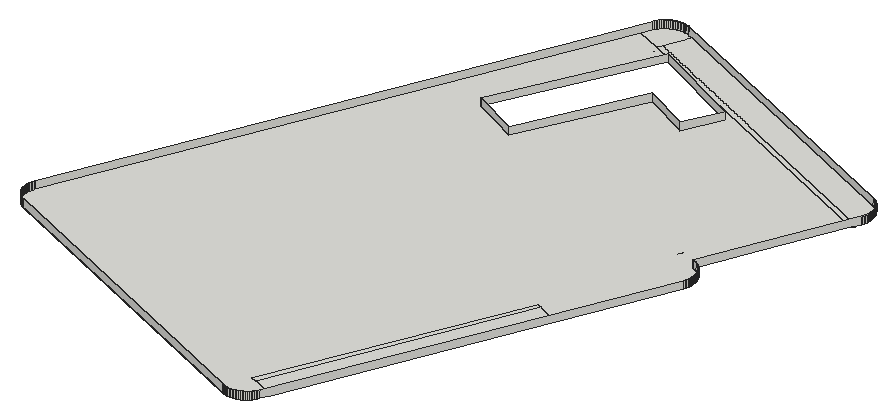
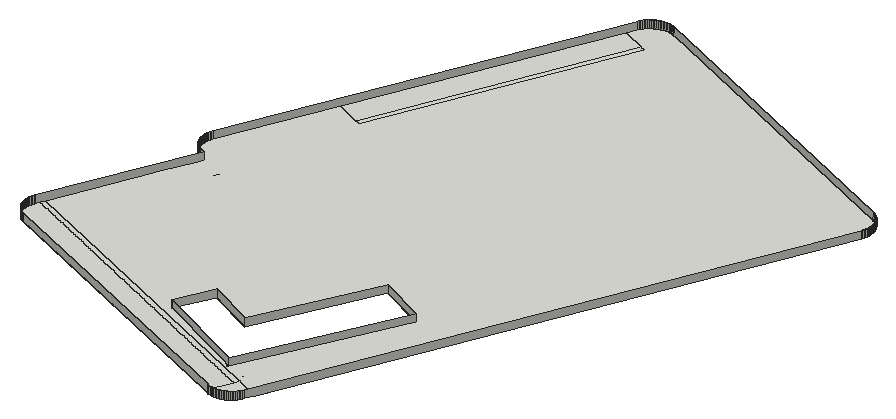
# SketchUp Ruby script. Lengths in inches.
U = 1.inch
M = Sketchup.active_model
def pt(a) = Geom::Point3d.new(a.map { |v| v * U })
def face(e, loops, mat)
  f = e.add_face(loops[0].map { |a| pt(a) })
  loops[1..].each { |l| e.add_face(l.map { |a| pt(a) }).erase! }
  f.material = f.back_material = mat if mat
  f
end
# faces: each face lists its corners as indices into pts; further lists are holes
def faces(e, pts, list, mat = nil) = list.each { |f| face(e, (f[0].is_a?(Array) ? f : [f]).map { |l| l.map { |i| pts[i] } }, mat) }
# xy, xz, yz: faces in a plane at the given z, y or x. An outline is a flat list of corners, or four numbers for a rectangle; further outlines are holes
def ring(l) = l.size == 4 ? [[l[0], l[1]], [l[2], l[1]], [l[2], l[3]], [l[0], l[3]]] : l.each_slice(2).to_a
def flat(e, list, mat, &to3) = list.each { |f| face(e, (f[0].is_a?(Array) ? f : [f]).map { |l| ring(l).map { |u, v| to3.(u, v) } }, mat) }
def xy(e, z, list, mat = nil) = flat(e, list, mat) { |x, y| [x, y, z] }
def xz(e, y, list, mat = nil) = flat(e, list, mat) { |x, z| [x, y, z] }
def yz(e, x, list, mat = nil) = flat(e, list, mat) { |y, z| [x, y, z] }
def lines(e, pts, list) = list.each { |a, b| e.add_line(pt(pts[a]), pt(pts[b])) }
# prism: a flat outline (further loops are holes) pulled along v
def prism(e, loops, v, mat = nil)
  f = face(e, loops, mat); d = Geom::Vector3d.new(v.map { |x| x * U })
  f.pushpull(f.normal.samedirection?(d) ? d.length : -d.length)
end
def box(e, o, s, mat = nil) = prism(e, [[o, [o[0] + s[0], o[1], o[2]], [o[0] + s[0], o[1] + s[1], o[2]], [o[0], o[1] + s[1], o[2]]]], [0, 0, s[2]], mat)
def at(x, y, z, deg = 0) = Geom::Transformation.translation(pt([x, y, z])) * Geom::Transformation.rotation(ORIGIN, Z_AXIS, deg.degrees)
def axes(o, x, y, z) = Geom::Transformation.new([*x, 0, *y, 0, *z, 0, *pt(o).to_a, 1])
def part(name) = M.definitions.add(name)
# library, detail: a bought-in or finely detailed component or shape, given as its bounding box
def library(name, o, s) = part(name).tap { |d| box(d.entities, o, s) }
def detail(e, o, s) = box(e.add_group.entities, o, s)
def put(e, d, t, mat = nil) = e.add_instance(d, t).tap { |i| i.material = mat if mat }
def group(e, t, mat = nil) = e.add_group.tap { |g| g.transformation = t; g.material = mat if mat }.entities
root = M.entities
xy(root,306,[[841.44,516.19,840.14,516.26,838.84,516.41,837.55,516.64,836.28,516.96,835.03,517.37,833.82,517.85,548.6875,642.03,547.51,642.59,546.36,643.23,545.26,643.94,544.21,644.73,543.22,645.57,542.28,646.49,541.4,647.46,540.59,648.48,539.85,649.56,539.18,650.68,538.58,651.85,538.0625,653.05,537.62,654.28,537.26,655.54,536.99,656.82,536.8,658.12,536.7,659.42,536.68,660.73,536.74,662.04,536.9,663.34,537.13,664.625,537.45,665.89,537.85,667.14,538.34,668.36,737.58,1125.82,759.58,1116.24,781.77,1106.57,780.33,1103.61,714.3125,967.65,757.25,946.81,807.7,1050.72,850.64,1029.87,866.2,1061.92,780.33,1103.61,781.77,1106.57,1037.38,995.25,1022.45,960.98,1002.39,914.92,999.84,909.07,987.46,880.65,985.47,876.0625,989.14,874.47,990.32,873.91,991.46,873.27,992.56,872.56,993.61,871.78,994.61,870.93,995.54,870.01,996.42,869.04,997.23,868.02,997.98,866.94,998.65,865.82,999.24,864.65,999.76,863.45,1000.2,862.22,1000.56,860.96,1000.83,859.68,1001.02,858.38,1001.13,857.08,1001.15,855.77,1001.08,854.46,1000.93,853.16,1000.69,851.875,1000.37,850.61,999.97,849.36,999.49,848.14,957.56,751.88,935.56,761.46,930.97,763.46,837.14,548.01,841.72,546.01,863.72,536.43,860.14,528.2,859.58,527.02,858.94,525.875,858.23,524.78,857.45,523.73,856.6,522.73,855.6875,521.79,854.72,520.91,853.69,520.1,852.61,519.36,851.49,518.6875,850.32,518.09,849.125,517.57,847.89,517.14,846.63,516.78,845.35,516.5,844.06,516.3125,842.75,516.21],[863.72,536.43,841.72,546.01,935.56,761.46,957.56,751.88],[841.72,546.01,837.14,548.01,930.97,763.46,935.56,761.46],[1037.38,995.25,781.77,1106.57,759.58,1116.24,761.77,1120.74,1039.375,999.83],[1037.38,995.25,1039.5625,999.75,1039.375,999.83],
  [1039.375,999.83,761.77,1120.74,771.35,1142.74,1030.62,1029.82,1031.8,1029.26,1032.95,1028.625,1034.04,1027.91,1035.09,1027.13,1036.09,1026.28,1037.03,1025.37,1037.91,1024.4,1038.72,1023.375,1039.46,1022.3,1040.13,1021.17,1040.73,1020.01,1041.25,1018.81,1041.6875,1017.57,1042.04,1016.31,1042.32,1015.03,1042.51,1013.74,1042.61,1012.44,1042.63,1011.125,1042.57,1009.82,1042.41,1008.52,1042.18,1007.23,1041.86,1005.96,1041.45,1004.72,1040.97,1003.5],[759.58,1116.24,737.58,1125.82,741.17,1134.07,741.73,1135.26,742.37,1136.4,743.08,1137.5,743.86,1138.55,744.71,1139.54,745.625,1140.48,746.59,1141.36,747.62,1142.17,748.7,1142.92,749.82,1143.59,750.99,1144.18,752.1875,1144.7,753.42,1145.14,754.68,1145.5,755.96,1145.77,757.26,1145.96,758.56,1146.07,759.87,1146.08,761.18,1146.02,762.48,1145.87,763.76,1145.63,765.03,1145.31,766.28,1144.91,767.49,1144.42,771.35,1142.74,761.77,1120.74]])
p = [[841.44,516.19,306],[841.44,516.19,312.91],[840.14,516.26,312.91],[840.14,516.26,306],[842.75,516.21,306],[842.75,516.21,312.91],
  [844.06,516.3125,306],[844.06,516.3125,312.91],[838.84,516.41,312.91],[838.84,516.41,306],[845.35,516.5,306],[845.35,516.5,312.91],
  [837.55,516.64,312.91],[837.55,516.64,306],[846.63,516.78,306],[846.63,516.78,312.91],[836.28,516.96,312.91],[836.28,516.96,306],
  [847.89,517.14,306],[847.89,517.14,312.91],[835.03,517.37,312.91],[835.03,517.37,306],[849.125,517.57,306],[849.125,517.57,312.91],
  [833.82,517.85,312.91],[833.82,517.85,306],[850.32,518.09,306],[850.32,518.09,312.91],[548.6875,642.03,312.91],[548.6875,642.03,306],
  [851.49,518.6875,306],[851.49,518.6875,312.91],[852.61,519.36,306],[852.61,519.36,312.91],[853.69,520.1,306],[853.69,520.1,312.91],
  [854.72,520.91,306],[854.72,520.91,312.91],[855.6875,521.79,306],[855.6875,521.79,312.91],[856.6,522.73,306],[856.6,522.73,312.91],
  [857.45,523.73,306],[857.45,523.73,312.91],[858.23,524.78,306],[858.23,524.78,312.91],[858.94,525.875,306],[858.94,525.875,312.91],
  [859.58,527.02,306],[859.58,527.02,312.91],[860.14,528.2,306],[860.14,528.2,312.91],[957.56,751.88,306],[999.49,848.14,306],
  [999.49,848.14,312.91],[863.72,536.43,306],[547.51,642.59,312.91],[547.51,642.59,306],[546.36,643.23,312.91],[546.36,643.23,306],
  [545.26,643.94,312.91],[545.26,643.94,306],[544.21,644.73,312.91],[544.21,644.73,306],[543.22,645.57,312.91],[543.22,645.57,306],
  [542.28,646.49,312.91],[542.28,646.49,306],[541.4,647.46,312.91],[541.4,647.46,306],[540.59,648.48,312.91],[540.59,648.48,306],
  [539.85,649.56,312.91],[539.85,649.56,306],[539.18,650.68,312.91],[539.18,650.68,306],[538.58,651.85,312.91],[538.58,651.85,306],
  [538.0625,653.05,312.91],[538.0625,653.05,306],[537.62,654.28,312.91],[537.62,654.28,306],[537.26,655.54,312.91],[537.26,655.54,306],
  [536.99,656.82,312.91],[536.99,656.82,306],[536.8,658.12,312.91],[536.8,658.12,306],[536.7,659.42,312.91],[536.7,659.42,306],
  [536.68,660.73,312.91],[536.68,660.73,306],[536.74,662.04,312.91],[536.74,662.04,306],[536.9,663.34,312.91],[536.9,663.34,306],
  [537.13,664.625,312.91],[537.13,664.625,306],[537.45,665.89,312.91],[537.45,665.89,306],[537.85,667.14,312.91],[537.85,667.14,306],
  [538.34,668.36,312.91],[538.34,668.36,306],[741.17,1134.07,312.91],[741.17,1134.07,306],[737.58,1125.82,306],[999.97,849.36,306],
  [999.97,849.36,312.91],[1000.37,850.61,306],[1000.37,850.61,312.91],[1000.69,851.875,306],[1000.69,851.875,312.91],[1000.93,853.16,306],
  [1000.93,853.16,312.91],[1001.08,854.46,306],[1001.08,854.46,312.91],[1001.15,855.77,306],[1001.15,855.77,312.91],[1001.13,857.08,306],
  [1001.13,857.08,312.91],[1001.02,858.38,306],[1001.02,858.38,312.91],[1000.83,859.68,306],[1000.83,859.68,312.91],[1000.56,860.96,306],
  [1000.56,860.96,312.91],[1000.2,862.22,306],[1000.2,862.22,312.91],[999.76,863.45,306],[999.76,863.45,312.91],[999.24,864.65,306],
  [999.24,864.65,312.91],[998.65,865.82,306],[998.65,865.82,312.91],[997.98,866.94,306],[997.98,866.94,312.91],[997.23,868.02,306],
  [997.23,868.02,312.91],[996.42,869.04,306],[996.42,869.04,312.91],[995.54,870.01,306],[995.54,870.01,312.91],[994.61,870.93,306],
  [994.61,870.93,312.91],[993.61,871.78,306],[993.61,871.78,312.91],[992.56,872.56,306],[992.56,872.56,312.91],[991.46,873.27,306],
  [991.46,873.27,312.91],[990.32,873.91,306],[990.32,873.91,312.91],[989.14,874.47,306],[989.14,874.47,312.91],[985.47,876.0625,312.91],
  [985.47,876.0625,306],[1039.375,999.83,306],[1040.97,1003.5,306],[1040.97,1003.5,312.91],[987.46,880.65,306],[999.84,909.07,306],
  [1002.39,914.92,306],[1022.45,960.98,306],[1037.38,995.25,306],[714.3125,967.65,312.91],[757.25,946.81,312.91],[757.25,946.81,306],
  [714.3125,967.65,306],[807.7,1050.72,312.91],[807.7,1050.72,306],[780.33,1103.61,312.91],[780.33,1103.61,306],[1041.45,1004.72,306],
  [1041.45,1004.72,312.91],[1041.86,1005.96,306],[1041.86,1005.96,312.91],[1042.18,1007.23,306],[1042.18,1007.23,312.91],[1042.41,1008.52,306],
  [1042.41,1008.52,312.91],[1042.57,1009.82,306],[1042.57,1009.82,312.91],[1042.63,1011.125,306],[1042.63,1011.125,312.91],[1042.61,1012.44,306],
  [1042.61,1012.44,312.91],[1042.51,1013.74,306],[1042.51,1013.74,312.91],[1042.32,1015.03,306],[1042.32,1015.03,312.91],[1042.04,1016.31,306],
  [1042.04,1016.31,312.91],[1041.6875,1017.57,306],[1041.6875,1017.57,312.91],[1041.25,1018.81,306],[1041.25,1018.81,312.91],[1040.73,1020.01,306],
  [1040.73,1020.01,312.91],[1040.13,1021.17,306],[1040.13,1021.17,312.91],[1039.46,1022.3,306],[1039.46,1022.3,312.91],[1038.72,1023.375,306],
  [1038.72,1023.375,312.91],[1037.91,1024.4,306],[1037.91,1024.4,312.91],[1037.03,1025.37,306],[1037.03,1025.37,312.91],[1036.09,1026.28,306],
  [1036.09,1026.28,312.91],[1035.09,1027.13,306],[1035.09,1027.13,312.91],[1034.04,1027.91,306],[1034.04,1027.91,312.91],[1032.95,1028.625,306],
  [1032.95,1028.625,312.91],[1031.8,1029.26,306],[1031.8,1029.26,312.91],[1030.62,1029.82,306],[1030.62,1029.82,312.91],[767.49,1144.42,312.91],
  [771.35,1142.74,306],[767.49,1144.42,306],[850.64,1029.87,312.91],[850.64,1029.87,306],[866.2,1061.92,306],[866.2,1061.92,312.91],
  [741.73,1135.26,312.91],[741.73,1135.26,306],[742.37,1136.4,312.91],[742.37,1136.4,306],[743.08,1137.5,312.91],[743.08,1137.5,306],
  [743.86,1138.55,312.91],[743.86,1138.55,306],[744.71,1139.54,312.91],[744.71,1139.54,306],[745.625,1140.48,312.91],[745.625,1140.48,306],
  [746.59,1141.36,312.91],[746.59,1141.36,306],[747.62,1142.17,312.91],[747.62,1142.17,306],[748.7,1142.92,312.91],[748.7,1142.92,306],
  [749.82,1143.59,312.91],[749.82,1143.59,306],[750.99,1144.18,312.91],[750.99,1144.18,306],[752.1875,1144.7,312.91],[752.1875,1144.7,306],
  [766.28,1144.91,306],[766.28,1144.91,312.91],[753.42,1145.14,312.91],[753.42,1145.14,306],[765.03,1145.31,306],[765.03,1145.31,312.91],
  [754.68,1145.5,312.91],[754.68,1145.5,306],[763.76,1145.63,306],[763.76,1145.63,312.91],[755.96,1145.77,312.91],[755.96,1145.77,306],
  [762.48,1145.87,306],[762.48,1145.87,312.91],[757.26,1145.96,312.91],[757.26,1145.96,306],[761.18,1146.02,306],[761.18,1146.02,312.91],
  [758.56,1146.07,312.91],[758.56,1146.07,306],[759.87,1146.08,306],[759.87,1146.08,312.91],[762.25,1109.625,306],[762.28,1109.71,306],
  [879.58,1064.05,306],[879.59,1064.06,306],[965.83,890.07,306],[963.48,885.23,306]]
faces(root,p,[[0,1,2,3],[4,5,1,0],[6,7,5,4],[3,2,8,9],[10,11,7,6],[9,8,12,13],[14,15,11,10],[13,12,16,17],
  [18,19,15,14],[17,16,20,21],[22,23,19,18],[21,20,24,25],[26,27,23,22],[24,28,29,25],[30,31,27,26],[32,33,31,30],
  [34,35,33,32],[36,37,35,34],[38,39,37,36],[40,41,39,38],[42,43,41,40],[44,45,43,42],[46,47,45,44],[48,49,47,46],
  [50,51,49,48],[52,53,54,51,50,55],[56,57,29,28],[58,59,57,56],[60,61,59,58],[62,63,61,60],[64,65,63,62],[66,67,65,64],
  [68,69,67,66],[70,71,69,68],[72,73,71,70],[74,75,73,72],[76,77,75,74],[78,79,77,76],[80,81,79,78],[82,83,81,80],
  [84,85,83,82],[86,87,85,84],[88,89,87,86],[90,91,89,88],[92,93,91,90],[94,95,93,92],[96,97,95,94],[98,99,97,96],
  [100,101,99,98],[102,103,101,100],[102,104,105,106,103],[54,53,107,108],[108,107,109,110],[110,109,111,112],[112,111,113,114],[114,113,115,116],
  [116,115,117,118],[118,117,119,120],[120,119,121,122],[122,121,123,124],[124,123,125,126],[126,125,127,128],[128,127,129,130],[130,129,131,132],
  [132,131,133,134],[134,133,135,136],[136,135,137,138],[138,137,139,140],[140,139,141,142],[142,141,143,144],[144,143,145,146],[146,145,147,148],
  [148,147,149,150],[150,149,151,152],[152,151,153,154],[155,154,153,156],[157,158,159,155,156,160,161,162,163,164],[165,166,167,168],[166,169,170,167],[171,165,168,172],
  [173,174,159,158],[175,176,174,173],[177,178,176,175],[179,180,178,177],[181,182,180,179],[183,184,182,181],[185,186,184,183],[187,188,186,185],
  [189,190,188,187],[191,192,190,189],[193,194,192,191],[195,196,194,193],[197,198,196,195],[199,200,198,197],[201,202,200,199],[203,204,202,201],
  [205,206,204,203],[207,208,206,205],[209,210,208,207],[211,212,210,209],[213,214,212,211],[215,216,214,213],[217,218,216,215],[219,220,218,217],
  [221,220,219,222,223],[224,225,170,169],[226,225,224,227],[227,171,172,226],[228,229,105,104],[230,231,229,228],[232,233,231,230],[234,235,233,232],
  [236,237,235,234],[238,239,237,236],[240,241,239,238],[242,243,241,240],[244,245,243,242],[246,247,245,244],[248,249,247,246],[250,251,249,248],
  [221,223,252,253],[254,255,251,250],[253,252,256,257],[258,259,255,254],[257,256,260,261],[262,263,259,258],[261,260,264,265],[266,267,263,262],
  [265,264,268,269],[270,271,267,266],[269,268,272,273],[273,272,271,270]])
lines(root,p,[[274,275],[276,277],[278,279]])
